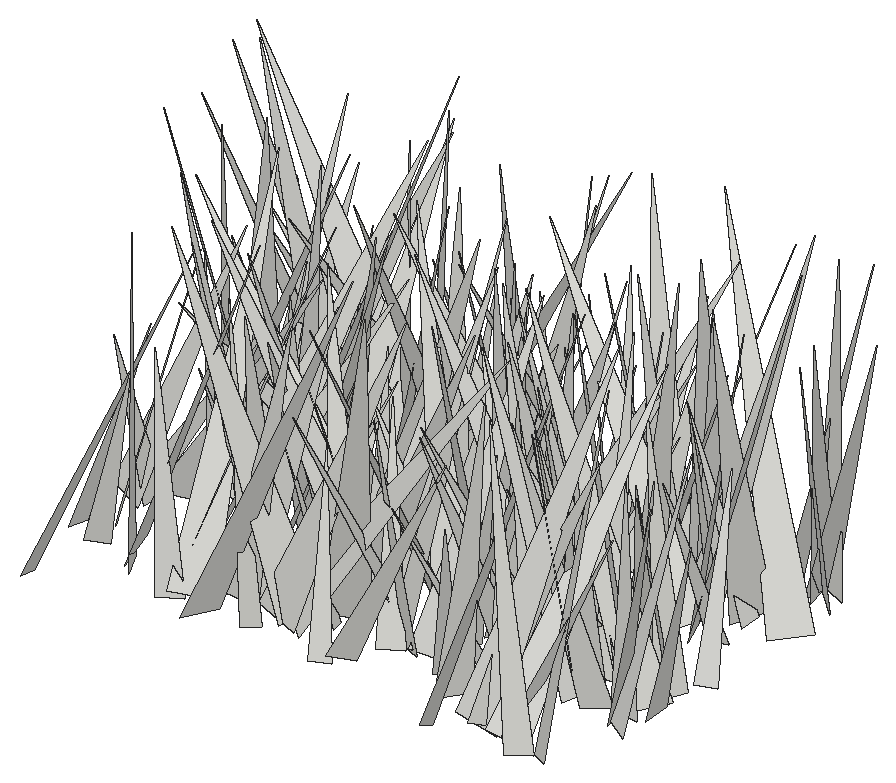
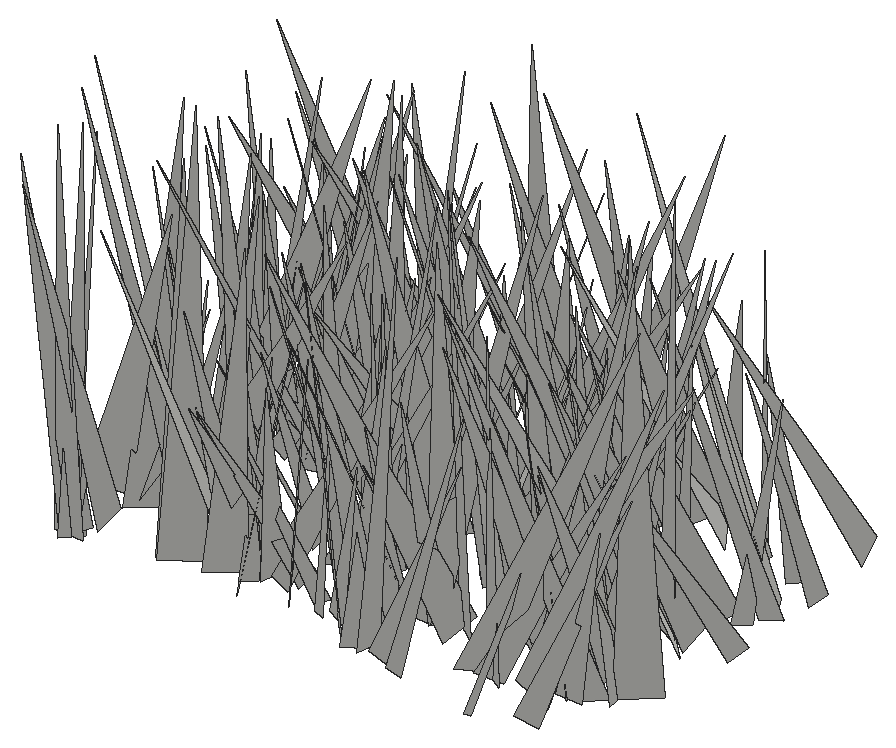
# SketchUp Ruby script. Lengths in inches.
U = 1.inch
M = Sketchup.active_model
def pt(a) = Geom::Point3d.new(a.map { |v| v * U })
def face(e, loops, mat)
  f = e.add_face(loops[0].map { |a| pt(a) })
  loops[1..].each { |l| e.add_face(l.map { |a| pt(a) }).erase! }
  f.material = f.back_material = mat if mat
  f
end
# faces: each face lists its corners as indices into pts; further lists are holes
def faces(e, pts, list, mat = nil) = list.each { |f| face(e, (f[0].is_a?(Array) ? f : [f]).map { |l| l.map { |i| pts[i] } }, mat) }
# xy, xz, yz: faces in a plane at the given z, y or x. An outline is a flat list of corners, or four numbers for a rectangle; further outlines are holes
def ring(l) = l.size == 4 ? [[l[0], l[1]], [l[2], l[1]], [l[2], l[3]], [l[0], l[3]]] : l.each_slice(2).to_a
def flat(e, list, mat, &to3) = list.each { |f| face(e, (f[0].is_a?(Array) ? f : [f]).map { |l| ring(l).map { |u, v| to3.(u, v) } }, mat) }
def xy(e, z, list, mat = nil) = flat(e, list, mat) { |x, y| [x, y, z] }
def xz(e, y, list, mat = nil) = flat(e, list, mat) { |x, z| [x, y, z] }
def yz(e, x, list, mat = nil) = flat(e, list, mat) { |y, z| [x, y, z] }
def lines(e, pts, list) = list.each { |a, b| e.add_line(pt(pts[a]), pt(pts[b])) }
# prism: a flat outline (further loops are holes) pulled along v
def prism(e, loops, v, mat = nil)
  f = face(e, loops, mat); d = Geom::Vector3d.new(v.map { |x| x * U })
  f.pushpull(f.normal.samedirection?(d) ? d.length : -d.length)
end
def box(e, o, s, mat = nil) = prism(e, [[o, [o[0] + s[0], o[1], o[2]], [o[0] + s[0], o[1] + s[1], o[2]], [o[0], o[1] + s[1], o[2]]]], [0, 0, s[2]], mat)
def at(x, y, z, deg = 0) = Geom::Transformation.translation(pt([x, y, z])) * Geom::Transformation.rotation(ORIGIN, Z_AXIS, deg.degrees)
def axes(o, x, y, z) = Geom::Transformation.new([*x, 0, *y, 0, *z, 0, *pt(o).to_a, 1])
def part(name) = M.definitions.add(name)
# library, detail: a bought-in or finely detailed component or shape, given as its bounding box
def library(name, o, s) = part(name).tap { |d| box(d.entities, o, s) }
def detail(e, o, s) = box(e.add_group.entities, o, s)
def put(e, d, t, mat = nil) = e.add_instance(d, t).tap { |i| i.material = mat if mat }
def group(e, t, mat = nil) = e.add_group.tap { |g| g.transformation = t; g.material = mat if mat }.entities
root = M.entities
c1 = part("fur_instance\#9")
p = [[0.8125,0,1.79],[0.67,-0.02,1.48],[0,-0.11,0],[0,0.11,0]]
faces(c1.entities,p,[[0,1,2,3]])
put(root,c1,axes([540.13,111.88,-21.66],[4.26333,-3.02404,0.31767],[-2.97687,-4.03955,1.49732],[0.61963,1.39963,5.00788]))
put(root,c1,axes([532.62,111.79,-21.86],[1.59272,-3.9303,2.28796],[-4.37909,-1.9795,-0.352],[-1.22702,1.96293,4.22612]))
put(root,c1,axes([548.95,110.64,-21.86],[-0.83276,5.81039,0.96307],[5.68734,0.54058,1.65638],[-1.53047,-1.15272,5.63121]))
put(root,c1,axes([534.11,111.59,-21.86],[7.97011,-1.5942,0.50435],[-1.65185,-7.88792,1.1707],[-0.25934,1.24806,8.04323]))
put(root,c1,axes([543.53,113.4375,-21.86],[1.84889,-3.8875,0.07331],[-3.87281,-1.83403,0.41727],[0.34554,0.24513,4.2845]))
put(root,c1,axes([544.58,112.5,-21.86],[5.43979,-3.16023,1.66658],[-3.30816,-5.60189,0.17546],[-1.34931,0.9938,6.28869]))
put(root,c1,axes([539.48,111.49,-21.86],[-1.47,3.64091,0.87512],[3.73843,1.4809,0.11844],[0.21496,-0.85654,3.92467]))
put(root,c1,axes([537.125,113.375,-21.66],[-7.26006,2.55391,1.83228],[2.95803,7.11093,1.80912],[1.0629,-2.34529,7.48051]))
put(root,c1,axes([538.2,114.54,-21.86],[5.23004,-6.31048,0.45418],[-6.32662,-5.22094,0.31214],[-0.04891,0.54893,8.19012]))
put(root,c1,axes([534.52,113.22,-21.86],[1.87666,-6.19619,1.68038],[-6.32701,-1.4881,1.57887],[1.08876,2.03251,6.27868]))
put(root,c1,axes([547.83,111.66,-21.86],[4.34496,-0.35551,0.43941],[-0.4633,-4.19131,1.19014],[-0.32376,1.22666,4.19388]))
put(root,c1,axes([527.7,110.08,-21.86],[6.20269,2.14266,0.41588],[1.88774,-5.89525,2.21806],[-1.09562,1.97291,6.17613]))
put(root,c1,axes([529.85,113.41,-21.66],[8.09633,1.85359,0.38508],[1.89305,-7.94545,-1.5559],[-0.02113,-1.6027,8.15877]))
put(root,c1,axes([536.59,112.72,-21.66],[1.17731,-6.81979,2.88625],[-6.91612,0.0321,2.89694],[2.64712,3.11697,6.28517]))
put(root,c1,axes([540.48,115.3,-21.86],[-4.62318,-3.47557,0.41553],[-3.19467,4.47097,1.85217],[1.4305,-1.24775,5.47931]))
put(root,c1,axes([528.21,113.3,-21.86],[2.52401,-3.24586,0.70539],[-3.32076,-2.44552,0.62916],[0.07602,0.94215,4.0633]))
put(root,c1,axes([546.7,111.22,-21.66],[3.7026,-0.58317,1.91769],[-1.4169,-3.61072,1.63767],[-1.41775,2.08554,3.37155]))
put(root,c1,axes([546.32,112.89,-21.86],[-2.72992,2.63061,1.69887],[2.87463,2.99911,-0.02472],[1.24209,-1.1593,3.79104]))
put(root,c1,axes([546.44,111.43,-21.86],[-0.17327,7.80384,1.95788],[7.72096,0.71202,-2.15474],[2.26272,-1.83203,7.50246]))
put(root,c1,axes([530.16,112.81,-21.86],[5.01686,3.02729,2.73746],[3.17963,-5.61852,0.38618],[-2.55892,-1.04628,5.84673]))
put(root,c1,axes([549.68,110.875,-21.86],[3.93388,5.26717,1.14139],[4.90502,-4.08461,1.94372],[-2.23307,0.30691,6.28017]))
put(root,c1,axes([545.24,113.75,-21.66],[1.83372,-5.8574,1.52699],[-5.60076,-1.03656,2.74963],[2.29617,2.14936,5.48737]))
put(root,c1,axes([543.79,115.04,-21.86],[-3.32799,-2.15223,0.18164],[-2.02775,3.22824,1.09879],[0.74386,-0.82886,3.80792]))
put(root,c1,axes([544.4,115.91,-21.86],[-5.45284,-1.57742,1.94379],[-0.6971,5.43147,2.45217],[2.40429,-2.00271,5.11943]))
put(root,c1,axes([549.77,115.1,-21.86],[5.98567,0.36805,0.66862],[0.55714,-5.71998,-1.83907],[-0.52163,-1.88604,5.70802]))
put(root,c1,axes([536.67,113.42,-21.86],[4.68753,6.76488,0.69054],[6.04009,-3.75687,-4.19721],[3.12373,-2.88717,7.07954]))
put(root,c1,axes([541.45,114.02,-21.86],[1.51862,3.68557,2.40948],[4.21899,-1.94756,0.31991],[-1.2606,-2.07817,3.97332]))
put(root,c1,axes([549,114.9,-21.86],[0.96308,-5.75121,1.64983],[-5.7805,-1.32563,-1.24675],[-1.54408,1.37555,5.69645]))
put(root,c1,axes([536.3125,111.65,-21.66],[-5.7713,0.32455,0.04644],[0.28097,5.31808,-2.2482],[0.16895,2.24233,5.3253]))
put(root,c1,axes([545.32,110.0625,-21.66],[6.83312,3.40706,1.30672],[2.45514,-6.34476,3.70451],[-2.69961,2.8536,6.67654]))
put(root,c1,axes([538.39,113.82,-21.86],[-3.92472,-1.58946,0.29836],[-1.61245,3.78584,-1.04222],[-0.12416,1.07696,4.10409]))
put(root,c1,axes([548.21,115.07,-21.66],[-6.07802,2.92755,1.98205],[3.37511,5.97833,1.51972],[1.05246,-2.26504,6.57292]))
put(root,c1,axes([534.47,113.95,-21.86],[0.67083,5.9533,2.27987],[6.17356,-0.03505,-1.72498],[1.58958,-2.37626,5.73727]))
put(root,c1,axes([526.89,113.92,-21.86],[4.46137,-0.22154,0.62784],[-0.29219,-4.4737,0.49769],[-0.59824,0.53291,4.43905]))
put(root,c1,axes([547.91,111.25,-21.86],[-2.00066,7.03095,0.19663],[6.73059,1.97306,-2.06922],[2.04255,0.38513,7.01108]))
put(root,c1,axes([540.86,113.7,-21.86],[-2.21571,3.96483,0.99922],[4.07213,2.24229,0.13245],[0.36886,-0.93805,4.54001]))
put(root,c1,axes([540.42,117.2,-21.86],[-2.55623,-6.61752,0.06611],[-6.61278,2.55692,0.25211],[0.25899,-0.02922,7.08959]))
put(root,c1,axes([546.97,116.01,-21.86],[3.91329,-2.80057,0.16354],[-2.76188,-3.89534,-0.61821],[-0.49189,-0.40864,4.7723]))
put(root,c1,axes([534.4,114.58,-21.66],[0.81184,5.62301,2.88886],[5.96448,-1.64652,1.52868],[-2.09495,-2.50871,5.47179]))
put(root,c1,axes([550.01,115.12,-21.86],[0.13174,-4.85064,1.64659],[-5.10405,0.01535,0.4536],[0.43432,1.65178,4.83118]))
put(root,c1,axes([533.375,116.34,-21.86],[3.50702,-4.68842,0.88051],[-4.69288,-3.58696,-0.4079],[-0.85643,0.45629,5.84073]))
put(root,c1,axes([538.15,116.29,-21.66],[-7.32197,2.2534,1.35544],[2.57225,6.97064,2.30649],[0.54639,-2.61889,7.30542]))
put(root,c1,axes([542.9,115.46,-21.86],[4.29298,-1.68508,0.76366],[-1.68331,-4.35833,-0.1541],[-0.76754,0.13347,4.60928]))
put(root,c1,axes([550.85,115.89,-21.86],[4.67229,-0.63233,0.28263],[-0.57173,-4.60903,-0.86025],[-0.39095,-0.81674,4.63574]))
put(root,c1,axes([541.96,117.6875,-21.86],[-3.16207,-7.07316,1.24758],[-6.76016,3.39142,2.09364],[2.42619,0.2311,7.45956]))
put(root,c1,axes([532.3125,112.21,-21.86],[5.9455,4.2001,0.21568],[4.05072,-5.81939,1.66213],[-1.13095,1.23699,7.08711]))
put(root,c1,axes([544.14,117.54,-21.66],[-5.03232,-2.4099,0.87584],[-1.92345,4.82363,2.22078],[1.6956,-1.68045,5.11859]))
put(root,c1,axes([550.45,114.18,-21.86],[2.85218,4.71528,1.10181],[4.83661,-2.83604,-0.38317],[-0.23454,-1.14272,5.49745]))
put(root,c1,axes([547.85,116.04,-21.86],[1.04102,-4.92803,1.21287],[-5.07408,-1.03535,0.14838],[-0.10125,1.21771,5.0346]))
put(root,c1,axes([546.28,116.83,-21.66],[-3.5454,-4.09399,1.47684],[-3.82101,3.83994,1.47185],[2.08366,0.07566,5.21193]))
put(root,c1,axes([547.375,116.23,-21.86],[-1.95958,-4.83915,1.26512],[-4.97855,2.01787,0.00704],[0.48156,1.1699,5.22085]))
put(root,c1,axes([534.35,115.44,-21.86],[-1.49858,-3.44059,1.04989],[-3.40031,0.98374,-1.62968],[-1.17382,1.54281,3.38047]))
put(root,c1,axes([527.92,116.85,-21.86],[-3.46561,0.71078,2.1355],[1.4755,3.67824,1.17025],[1.69955,-1.74395,3.33859]))
put(root,c1,axes([537.96,114.9,-21.86],[2.97491,-4.25566,3.74848],[-5.0806,-3.88069,-0.37363],[-2.51977,2.80026,5.17891]))
put(root,c1,axes([545.91,116.07,-21.86],[-5.4764,4.5647,2.90915],[5.14181,5.68019,0.76664],[1.69155,-2.48788,7.08799]))
put(root,c1,axes([533.31,112.08,-21.66],[-6.01479,5.28528,0.0687],[5.03484,5.76049,-2.36301],[1.60915,1.73181,7.65037]))
put(root,c1,axes([550.21,117.41,-21.86],[-3.52584,-3.38703,1.52089],[-2.9555,3.82986,1.67745],[2.24724,-0.27722,4.59235]))
put(root,c1,axes([549.83,115.68,-21.86],[-4.59653,-5.39297,2.39685],[-5.86856,4.49796,-1.13384],[0.62378,2.57709,6.99476]))
put(root,c1,axes([533.56,118.7,-21.66],[5.51839,-2.97407,0.09463],[-2.75984,-5.19025,-2.17974],[-1.11235,-1.87694,5.87762]))
put(root,c1,axes([550.38,116.03,-21.86],[-5.06971,5.94983,1.91077],[6.22333,4.58369,2.23904],[-0.56711,-2.88838,7.48926]))
put(root,c1,axes([536.01,117.22,-21.86],[-0.89834,-6.55906,1.37521],[-6.65422,0.70817,-0.96916],[-0.7961,1.48213,6.54897]))
put(root,c1,axes([527.68,115.08,-21.86],[4.69542,3.0157,0.91715],[3.05189,-4.76105,0.03053],[-0.78841,-0.46959,5.58037]))
put(root,c1,axes([533.8125,115.41,-21.66],[0.77097,6.55392,2.92574],[6.60675,-1.79779,2.28627],[-2.8044,-2.43357,6.19042]))
put(root,c1,axes([548.8,117.91,-21.66],[5.13341,-1.95182,0.40555],[-1.78394,-4.9977,-1.47188],[-0.88973,-1.24068,5.29103]))
put(root,c1,axes([537.57,116.55,-21.86],[5.33015,-4.46349,0.382],[-4.4244,-5.15196,1.5366],[0.7024,1.41905,6.78027]))
put(root,c1,axes([536.43,118.1,-21.86],[-3.15103,-4.03715,0.66571],[-3.75697,3.18756,1.54769],[1.62077,-0.46003,4.88182]))
put(root,c1,axes([542.21,114.17,-21.86],[-2.57926,6.41675,1.59968],[6.21683,2.93816,-1.76197],[2.25493,-0.76079,6.68751]))
put(root,c1,axes([549.9,115.4,-21.86],[-3.7674,-0.4134,0.34529],[-0.49063,3.64055,-0.99453],[0.22227,1.02903,3.6572]))
put(root,c1,axes([546.09,117.62,-21.86],[2.81422,-5.9892,1.8303],[-5.99838,-3.15452,-1.09945],[-1.79999,1.14839,6.52546]))
put(root,c1,axes([542.93,118.09,-21.86],[2.46673,-5.38252,0.46134],[-5.39282,-2.42347,0.55987],[0.31917,0.65147,5.89431]))
put(root,c1,axes([527.09,116.24,-21.66],[1.94999,6.06367,1.85826],[6.06829,-1.21894,-2.39034],[1.84311,-2.40204,5.90397]))
put(root,c1,axes([531.21,116.1,-21.86],[1.89742,4.59885,2.05217],[4.78177,-2.33318,0.8074],[-1.57969,-1.53878,4.90894]))
put(root,c1,axes([547.84,117.59,-21.66],[-0.53868,-3.7535,0.51973],[-3.36849,0.23389,-1.80211],[-1.73555,0.71104,3.33637]))
put(root,c1,axes([546.92,116.97,-21.86],[-4.89111,-2.11302,1.38613],[-2.21595,5.03778,-0.13961],[1.21481,0.68196,5.3262]))
put(root,c1,axes([534.68,116,-21.86],[3.00056,3.161,0.00616],[3.13284,-2.97269,-0.58633],[0.42105,-0.40809,4.31874]))
put(root,c1,axes([543.22,116.77,-21.86],[4.40781,-2.35415,1.32075],[-2.57038,-4.43283,0.67704],[-0.82436,1.23418,4.95101]))
put(root,c1,axes([537.49,117.17,-21.66],[-6.42815,4.45601,0.04956],[4.21627,6.0534,2.59983],[-1.44275,-2.16333,7.37686]))
put(root,c1,axes([534.27,116.5,-21.86],[-6.33694,-5.31771,1.42218],[-5.44687,5.74429,-2.79146],[-0.79519,3.03026,7.78734]))
put(root,c1,axes([548.55,117.42,-21.86],[4.13906,-0.88394,1.08396],[-0.87234,-4.27812,-0.15771],[-1.09332,0.06702,4.22946]))
put(root,c1,axes([550.51,117.13,-21.86],[-4.8782,2.33838,1.88669],[2.5546,5.12175,0.25721],[1.58166,-1.06025,5.40358]))
put(root,c1,axes([540.54,117.47,-21.86],[-3.99734,1.08155,0.32432],[1.12476,3.91891,0.79421],[0.09918,-0.85212,4.0642]))
put(root,c1,axes([540.3,114.92,-21.86],[3.95249,6.61953,0.92655],[6.54498,-4.05132,1.02412],[-1.35642,-0.25967,7.64143]))
put(root,c1,axes([538.4,116.52,-21.86],[0.74046,6.81709,2.01452],[6.9144,-0.22063,-1.79488],[1.64984,-2.13492,6.61811]))
put(root,c1,axes([541.99,118.81,-21.86],[-0.40221,-7.56998,1.93164],[-7.73436,0.65878,0.97125],[1.10251,1.85984,7.51818]))
put(root,c1,axes([533.27,117.26,-21.86],[3.86213,1.08614,0.2172],[1.09096,-3.86634,-0.0646],[-0.19154,-0.12107,4.01143]))
put(root,c1,axes([547.66,119.05,-21.86],[-2.21382,-3.77344,0.32599],[-3.76288,2.23425,0.30817],[0.43109,0.1241,4.36404]))
put(root,c1,axes([528.39,117.23,-21.66],[4.87522,-3.55324,0.35007],[-3.38958,-4.41978,2.34354],[1.12198,2.08707,5.55888]))
put(root,c1,axes([537.9,116.41,-21.86],[-1.59343,4.55905,1.08338],[4.45907,1.82697,-1.12985],[1.44061,-0.61229,4.69546]))
put(root,c1,axes([544.08,116.91,-21.86],[-4.34264,3.05124,0.46122],[3.07623,4.34339,0.23041],[0.24406,-0.45414,5.3024]))
put(root,c1,axes([544.53,118.43,-21.66],[-6.88709,2.46248,0.81316],[2.58785,6.67518,1.70354],[0.16756,-1.88022,7.11293]))
put(root,c1,axes([547.6,117.21,-21.86],[-0.37721,6.24874,2.25952],[6.16262,-0.51732,2.45945],[-2.4848,-2.23161,5.75674]))
put(root,c1,axes([533.16,118.85,-21.86],[7.51831,-0.309,0.51299],[-0.23256,-7.46002,-1.08516],[-0.55186,-1.06592,7.446]))
put(root,c1,axes([529.46,119.04,-21.86],[-3.84702,-6.56229,2.86732],[-6.71624,4.43571,1.14075],[2.48541,1.82909,7.52076]))
put(root,c1,axes([541.1,116.99,-21.86],[2.27452,-5.56414,4.58515],[-6.58849,-3.55674,-1.04785],[-2.92831,3.68058,5.91904]))
put(root,c1,axes([543.28,117.01,-21.86],[4.54007,-1.04122,1.07478],[-1.33062,-4.37982,1.37772],[-0.68465,1.60765,4.44952]))
put(root,c1,axes([531.35,115.93,-21.66],[3.64416,1.65962,0.06909],[1.4569,-3.27351,1.789],[-0.79783,1.60274,3.58241]))
put(root,c1,axes([547.92,116.71,-21.86],[0.35449,6.1752,1.09899],[6.2119,-0.49795,0.79425],[-0.86782,-1.04187,6.13416]))
put(root,c1,axes([531.64,117.625,-21.86],[2.64561,4.33348,1.24236],[4.47199,-2.70465,-0.08904],[-0.56902,-1.10798,5.07645]))
put(root,c1,axes([536.91,119.99,-21.86],[-3.28468,-3.33783,0.1825],[-3.30088,3.27904,0.56182],[0.52783,-0.26523,4.64915]))
put(root,c1,axes([539.6,118.23,-21.86],[3.87683,-5.48097,2.21285],[-5.90731,-3.50163,1.67625],[0.20355,2.76859,6.50085]))
put(root,c1,axes([531.17,117.83,-21.66],[2.97178,5.39968,0.42783],[5.06638,-2.59832,-2.39825],[1.91609,-1.5044,5.67771]))
put(root,c1,axes([535.83,119.92,-21.66],[4.04324,-6.81137,0.9787],[-6.74817,-3.70246,2.11055],[1.34718,1.89668,7.63467]))
put(root,c1,axes([531.83,119.96,-21.86],[3.06125,-3.87557,0.82155],[-3.90702,-3.12527,-0.1848],[-0.65588,0.52812,4.93529]))
put(root,c1,axes([541.24,116.11,-21.66],[5.35308,0.77922,1.1136],[0.09871,-4.73607,2.83947],[-1.35556,2.73224,4.60435]))
put(root,c1,axes([532.5,122.125,-21.86],[-5.57045,-1.42182,0.3414],[-1.0257,4.7578,3.07884],[1.04215,-2.91715,4.85512]))
put(root,c1,axes([533.02,121,-21.66],[7.23074,-0.77372,0.74856],[-0.57311,-7.06946,-1.77111],[-0.91134,-1.69312,7.05304]))
put(root,c1,axes([544.05,117.88,-21.86],[-4.80614,1.67739,0.07303],[1.63862,4.73444,-0.90443],[0.36591,0.83033,5.00945]))
put(root,c1,axes([550.97,118.46,-21.86],[-1.59242,3.59476,0.56652],[3.61736,1.63113,-0.18207],[0.39739,-0.44291,3.92746]))
put(root,c1,axes([535.79,119.32,-21.86],[-2.47,2.58512,1.49197],[2.74392,2.72878,-0.18549],[1.17462,-0.93843,3.57063]))
put(root,c1,axes([526.6875,118.6,-21.86],[3.53802,-1.77872,0.68161],[-1.86523,-2.94336,2.00089],[0.38644,2.07817,3.41729]))
put(root,c1,axes([549.37,121.13,-21.86],[0.58704,-3.79537,0.45103],[-3.78334,-0.64184,-0.47675],[-0.5428,0.36891,3.81079]))
put(root,c1,axes([530.92,118.11,-21.66],[-0.22471,7.89617,1.63504],[7.5306,0.79034,-2.78188],[2.88322,-1.44886,7.39332]))
put(root,c1,axes([542.29,121.09,-21.86],[0.10364,-5.95888,1.80759],[-6.13378,0.21397,1.05707],[1.07352,1.79787,5.86529]))
put(root,c1,axes([536.6,123.51,-21.86],[-0.28609,-7.90952,0.17476],[-7.91116,0.28452,-0.07401],[-0.06767,0.17732,7.91434]))
put(root,c1,axes([528.54,118.65,-21.86],[6.82155,0.82248,0.97272],[0.53436,-6.65794,1.88216],[-1.15634,1.77527,6.60814]))
put(root,c1,axes([541.47,119.96,-21.86],[-4.67336,-1.61213,2.14084],[-2.03116,4.93814,-0.71533],[1.7483,1.42769,4.89159]))
put(root,c1,axes([545.96,121.4,-21.86],[6.97924,-1.80721,1.76653],[-1.77915,-7.19853,-0.33521],[-1.79479,0.10824,7.20163]))
put(root,c1,axes([530.98,121.05,-21.86],[6.1687,-0.67373,2.21616],[-0.70194,-6.55164,-0.0379],[-2.20738,0.2006,6.20527]))
put(root,c1,axes([539.13,123.33,-21.86],[-3.51133,-6.12863,1.17286],[-5.90116,3.69891,1.66117],[2.0278,0.152,6.86513]))
put(root,c1,axes([533.65,122.86,-21.66],[7.53646,1.85279,1.2332],[2.16443,-7.11553,-2.53698],[-0.51849,-2.77277,7.33449]))
put(root,c1,axes([527.4375,123.11,-21.86],[5.72891,-5.77899,0.7373],[-5.79412,-5.75966,-0.12335],[-0.60698,0.43635,8.13646]))
put(root,c1,axes([528.52,119.61,-21.86],[3.1839,3.43631,0.24845],[3.39454,-3.18669,0.57383],[-0.5891,0.20968,4.64932]))
put(root,c1,axes([541.34,122.4375,-21.66],[-6.98354,0.71492,0.27676],[0.75932,6.7998,1.59491],[0.10557,-1.6153,6.83646]))
put(root,c1,axes([549.15,123.25,-21.86],[6.05759,-4.04132,1.47541],[-3.82561,-6.22554,-1.34569],[-1.96821,-0.33746,7.15653]))
put(root,c1,axes([548.12,121.49,-21.86],[7.78659,2.72532,1.24866],[2.87625,-7.77148,-0.97412],[-0.84485,-1.33952,8.19204]))
put(root,c1,axes([529.45,122.82,-21.86],[2.70621,-3.86796,1.26709],[-3.69816,-2.97221,-1.17466],[-1.70008,0.30833,4.57219]))
put(root,c1,axes([547.88,121.72,-21.86],[5.68987,2.39384,1.65752],[2.61602,-5.80047,-0.60296],[-1.2784,-1.21517,6.14342]))
put(root,c1,axes([542.3,120.1,-21.66],[3.82071,6.83533,0.31448],[6.59967,-3.58608,-2.23672],[1.80694,-1.35528,7.50444]))
put(root,c1,axes([543.85,120.84,-21.86],[1.90499,3.12749,0.05078],[3.06447,-1.8542,-0.76405],[0.62675,-0.43991,3.5814]))
put(root,c1,axes([536.86,122.01,-21.86],[-1.49682,6.02983,3.22428],[6.74332,1.8484,-0.32627],[1.1325,-3.03643,6.20426]))
put(root,c1,axes([546.71,122.23,-21.86],[-0.07394,-6.12578,2.47714],[-6.56947,-0.19789,-0.68546],[-0.70961,2.47033,6.08776]))
put(root,c1,axes([548.07,122.59,-21.86],[-1.67476,-3.89018,1.26522],[-4.03938,1.78862,0.15259],[0.64624,1.09838,4.23261]))
put(root,c1,axes([548.06,121.43,-21.66],[-5.28258,5.45364,0.12335],[5.18528,4.96674,2.47132],[-1.69419,-1.80343,7.17917]))
put(root,c1,axes([530.01,122.37,-21.86],[3.87779,-2.1954,0.31482],[-2.2129,-3.78759,0.8446],[0.14815,0.88911,4.37535]))
put(root,c1,axes([533.57,121.99,-21.86],[-3.36679,-6.63148,1.92496],[-6.20382,1.96447,-4.08298],[-3.03226,3.34389,6.21619]))
put(root,c1,axes([539.9,123.3125,-21.66],[2.36521,-5.47601,0.71506],[-5.30162,-2.03369,1.96193],[1.54624,1.40343,5.6331]))
put(root,c1,axes([531.82,118.87,-21.66],[7.42778,3.7642,0.92799],[3.25227,-7.14156,2.93652],[-2.11023,2.24305,7.79217]))
put(root,c1,axes([542.91,121.39,-21.86],[4.041,0.55824,1.1889],[0.26805,-4.11576,1.02147],[-1.28579,0.89645,3.94942]))
put(root,c1,axes([535.05,123.1875,-21.86],[-4.52397,-6.09316,3.51067],[-6.34353,5.33763,1.08955],[3.03497,2.07386,7.51038]))
put(root,c1,axes([549.375,122.9,-21.86],[-4.29082,0.07848,0.62907],[0.12494,4.3243,0.31276],[0.62151,-0.32753,4.28013]))
put(root,c1,axes([531.06,123.35,-21.86],[-7.80525,1.8691,2.4402],[2.24771,8.01322,1.05174],[2.09664,-1.63243,7.95672]))
put(root,c1,axes([541.05,121.73,-21.86],[-2.72966,-3.54913,3.67888],[-4.47058,3.67982,0.23296],[2.47878,2.72838,4.47136]))
put(root,c1,axes([539.53,121.52,-21.86],[-3.18847,2.06393,0.29466],[1.98964,3.17316,-0.69666],[0.62286,0.42918,3.73374]))
put(root,c1,axes([542.49,124.4,-21.86],[-1.24481,-6.10899,0.55091],[-5.80958,0.99391,-2.10566],[-1.96776,0.93016,5.86818]))
put(root,c1,axes([529.86,120.07,-21.86],[1.84381,6.83005,0.32521],[6.75707,-1.87158,0.99709],[-1.04756,-0.05069,7.00393]))
put(root,c1,axes([527.91,123.8,-21.86],[5.69454,1.71793,1.14191],[1.95584,-5.5622,-1.38552],[-0.6557,-1.67144,5.78441]))
put(root,c1,axes([537.625,124.17,-21.86],[5.69502,0.05498,1.49404],[0.36012,-5.7612,-1.16071],[-1.45103,-1.21405,5.57575]))
put(root,c1,axes([545.79,125.4,-21.86],[4.25947,-6.86655,0.67935],[-6.89421,-4.26807,0.08653],[-0.2843,0.62304,8.07992]))
put(root,c1,axes([546.07,125.31,-21.86],[3.44417,-6.15496,0.43731],[-6.17002,-3.42915,0.33004],[0.07525,0.54268,7.04535]))
put(root,c1,axes([538.05,121.47,-21.86],[2.63979,2.66437,0.28601],[2.37928,-2.51517,1.47039],[-1.23275,0.85099,3.4504]))
put(root,c1,axes([544.375,124.46,-21.66],[5.4983,0.81734,0.21266],[0.84397,-5.26527,-1.58403],[0.03145,-1.59793,5.32824]))
put(root,c1,axes([550.22,125.94,-21.86],[-3.37811,-5.89928,1.5704],[-5.1932,3.72048,2.80499],[3.2091,-0.18922,6.19235]))
put(root,c1,axes([547.1,123.24,-21.86],[-0.81294,-7.33898,4.00432],[-7.82592,2.08335,2.22952],[2.94113,3.51498,7.03923]))
put(root,c1,axes([536.1875,123.11,-21.86],[3.92282,-1.4058,1.44453],[-1.66907,-4.03753,0.60333],[-1.1301,1.0833,4.1232]))
put(root,c1,axes([543.11,125.07,-21.86],[3.64038,-1.44849,0.64201],[-1.22649,-3.59476,-1.15586],[-1.003,-0.8615,3.74359]))
put(root,c1,axes([543.15,123.89,-21.86],[4.61454,1.12705,1.27743],[1.23829,-4.75228,-0.2803],[-1.16993,-0.58453,4.7419]))
put(root,c1,axes([531.35,127.71,-21.86],[-5.60645,-3.595,0.79099],[-2.74257,5.04084,3.47133],[2.4552,-2.57833,5.68385]))
put(root,c1,axes([549.85,126.43,-21.86],[7.1612,-0.61813,1.17268],[-0.1707,-6.81898,-2.55193],[-1.31459,-2.48182,6.71956]))
put(root,c1,axes([529.51,124.63,-21.86],[3.73633,3.15118,1.53756],[3.50493,-3.41917,-1.50964],[-0.09758,-2.15258,4.64878]))
put(root,c1,axes([532.375,125.25,-21.86],[-4.08347,2.98679,1.40676],[3.27171,3.36098,2.36101],[-0.44252,-2.71247,4.47451]))
put(root,c1,axes([532,122.19,-21.66],[-2.25135,6.36064,1.32657],[6.19225,2.52565,-1.60099],[1.96812,-0.67041,6.55463]))
put(root,c1,axes([528.83,122.58,-21.66],[-4.17558,2.72173,1.55923],[2.19552,4.39009,-1.78362],[2.24025,0.77057,4.65424]))
put(root,c1,axes([537.99,123.02,-21.86],[0.78964,4.34465,0.57519],[4.335,-0.86018,0.54605],[-0.64386,-0.46311,4.38193]))
put(root,c1,axes([537.33,126.46,-21.86],[4.67947,-2.49587,0.44393],[-2.29207,-4.56374,-1.49753],[-1.08298,-1.12554,5.08765]))
put(root,c1,axes([528.54,124.1875,-21.86],[1.93796,6.92662,2.2466],[6.80944,-0.90011,-3.09877],[2.58009,-2.82714,6.49087]))
put(root,c1,axes([543.96,124.03,-21.86],[-1.54169,4.36128,2.00643],[4.43238,2.10262,-1.16464],[1.84406,-1.40768,4.47674]))
put(root,c1,axes([539.79,125.36,-21.86],[-1.86728,-3.21645,1.13397],[-3.16749,2.11482,0.78275],[1.26429,0.54787,3.63587]))
put(root,c1,axes([535.29,123.22,-21.86],[7.82793,-0.68601,0.13891],[-0.69946,-7.6099,1.83483],[0.02566,1.8399,7.64072]))
put(root,c1,axes([551.1,122.97,-21.86],[-3.56857,7.17935,0.49748],[7.02506,3.35468,1.97986],[-1.56176,-1.31463,7.76903]))
put(root,c1,axes([532.21,125.23,-21.86],[-3.26006,-5.04679,2.60885],[-5.29814,3.78652,0.70434],[2.05082,1.75965,5.96674]))
put(root,c1,axes([532.75,125.4,-21.66],[-7.09229,4.18803,1.11711],[4.32642,6.70959,2.31334],[-0.26383,-2.55536,7.90497]))
put(root,c1,axes([541.2,125.23,-21.86],[-3.54566,-2.66431,1.6705],[-2.78653,3.82874,0.19209],[1.45754,0.83849,4.43096]))
put(root,c1,axes([549.89,126.13,-21.86],[6.64533,-1.36705,0.39109],[-1.31179,-6.61549,-0.83466],[-0.54862,-0.74069,6.73295]))
put(root,c1,axes([536.72,126.45,-21.66],[6.67439,0.3641,2.55328],[0.99441,-6.8993,-1.61558],[-2.3797,-1.86182,6.48614]))
put(root,c1,axes([540.21,124.63,-21.86],[1.07989,-3.22676,1.49499],[-3.22529,-0.23045,1.83235],[1.49815,1.82977,2.86716]))
put(root,c1,axes([530.5,125.22,-21.86],[-0.67807,6.71445,3.30984],[6.96597,-0.65101,2.74773],[-2.74118,-3.31527,6.16389]))
put(root,c1,axes([538.54,122.29,-21.86],[4.01654,5.38759,0.39242],[5.219,-3.99648,1.45013],[-1.3936,0.56102,6.56169]))
put(root,c1,axes([537.26,125.53,-21.66],[0.1838,-6.38239,2.38865],[-6.46729,0.58989,2.0738],[2.14821,2.32195,6.03888]))
put(root,c1,axes([541.55,123.77,-21.86],[3.96425,-0.56902,0.64503],[-0.79665,-3.57598,1.74151],[-0.32433,1.82859,3.60641]))
put(root,c1,axes([536.32,126.48,-21.86],[-0.56318,-3.80765,0.20803],[-3.75255,0.51599,-0.71463],[-0.67806,0.30692,3.78215]))
put(root,c1,axes([529.21,127.13,-21.66],[1.40326,-4.201,0.43994],[-3.89786,-1.46649,-1.57071],[-1.62745,-0.10993,4.1413]))
put(root,c1,axes([543.14,125.61,-21.86],[-4.28874,-2.62611,1.19653],[-2.76089,4.3576,-0.33198],[0.84,0.91449,5.01792]))
put(root,c1,axes([535.1875,126.99,-21.86],[-1.82356,-4.42835,0.39133],[-4.41286,1.85435,0.42054],[0.53859,0.19978,4.77062]))
put(root,c1,axes([549.99,126.42,-21.86],[-1.4348,-7.0433,2.45033],[-7.23254,1.92235,1.29061],[1.81726,2.08982,7.07114]))
put(root,c1,axes([529.3,124.65,-21.86],[-1.4583,4.1794,0.64732],[4.14586,1.27741,1.09233],[-0.83566,-0.95598,4.28962]))
put(root,c1,axes([544.41,124.19,-21.86],[6.025,3.41302,0.55167],[3.40656,-6.04972,0.22351],[-0.59027,-0.07668,6.92094]))
put(root,c1,axes([542.66,124.1875,-21.86],[-4.55116,2.07867,0.64916],[1.93391,4.54938,-1.00919],[1.00113,0.66152,4.90056]))
put(root,c1,axes([544.15,125.1,-21.86],[-4.3858,5.26104,2.02142],[5.54364,4.48874,0.34523],[1.01623,-1.78118,6.84066]))
put(root,c1,axes([549.54,124.72,-21.86],[6.67173,1.075,1.66778],[0.88806,-6.84957,0.86244],[-1.77439,0.61387,6.70252]))
put(root,c1,axes([543.77,123.14,-21.86],[-3.94545,3.07895,0.18102],[2.74281,3.63702,-2.08047],[1.41057,1.53994,4.55172]))
put(root,c1,axes([538.35,125.96,-21.86],[-4.08433,-4.26667,3.28401],[-4.58243,4.91876,0.69141],[2.82675,1.80893,5.86585]))
put(root,c1,axes([539.09,125.24,-21.86],[0.66208,3.60921,1.19442],[3.54519,-1.02396,1.12897],[-1.37285,-0.90361,3.49144]))
